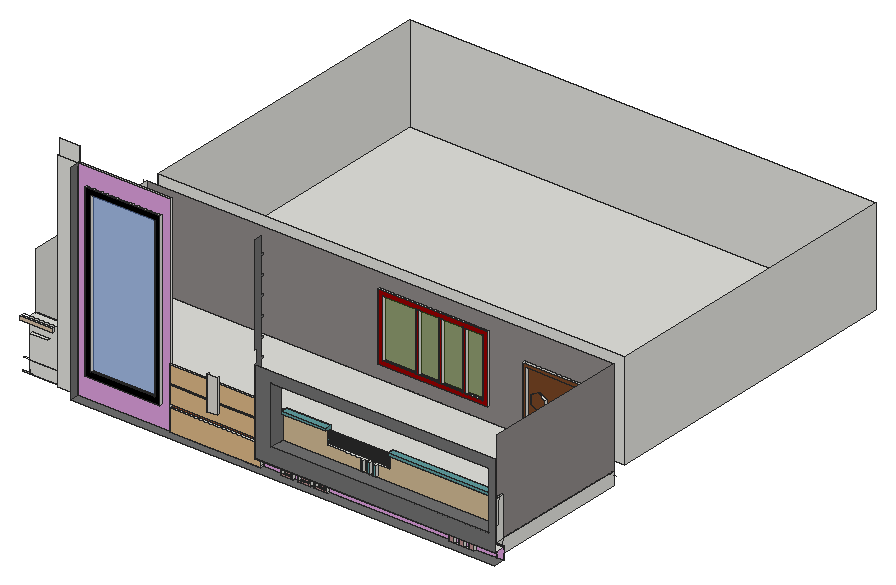
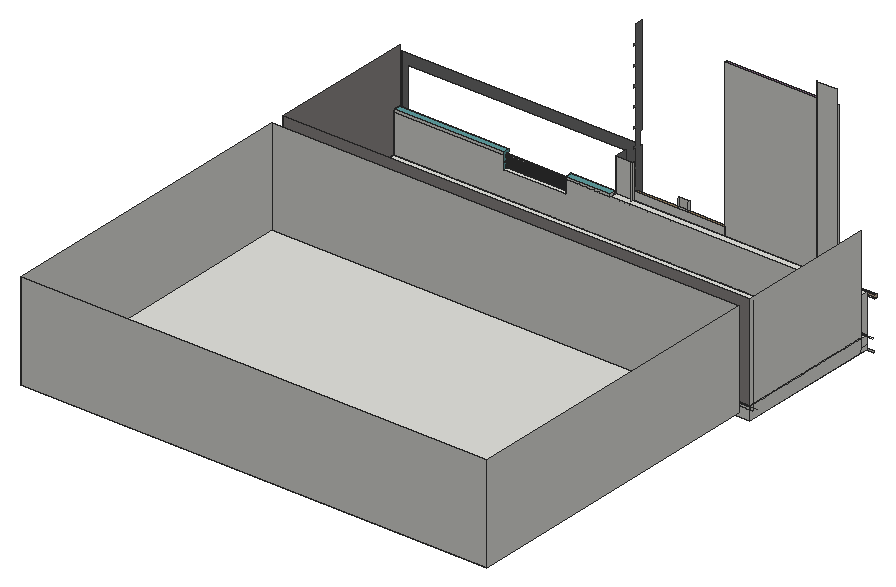
# SketchUp Ruby script. Lengths in inches.
U = 1.inch
M = Sketchup.active_model
def pt(a) = Geom::Point3d.new(a.map { |v| v * U })
def face(e, loops, mat)
  f = e.add_face(loops[0].map { |a| pt(a) })
  loops[1..].each { |l| e.add_face(l.map { |a| pt(a) }).erase! }
  f.material = f.back_material = mat if mat
  f
end
# faces: each face lists its corners as indices into pts; further lists are holes
def faces(e, pts, list, mat = nil) = list.each { |f| face(e, (f[0].is_a?(Array) ? f : [f]).map { |l| l.map { |i| pts[i] } }, mat) }
# xy, xz, yz: faces in a plane at the given z, y or x. An outline is a flat list of corners, or four numbers for a rectangle; further outlines are holes
def ring(l) = l.size == 4 ? [[l[0], l[1]], [l[2], l[1]], [l[2], l[3]], [l[0], l[3]]] : l.each_slice(2).to_a
def flat(e, list, mat, &to3) = list.each { |f| face(e, (f[0].is_a?(Array) ? f : [f]).map { |l| ring(l).map { |u, v| to3.(u, v) } }, mat) }
def xy(e, z, list, mat = nil) = flat(e, list, mat) { |x, y| [x, y, z] }
def xz(e, y, list, mat = nil) = flat(e, list, mat) { |x, z| [x, y, z] }
def yz(e, x, list, mat = nil) = flat(e, list, mat) { |y, z| [x, y, z] }
def lines(e, pts, list) = list.each { |a, b| e.add_line(pt(pts[a]), pt(pts[b])) }
# prism: a flat outline (further loops are holes) pulled along v
def prism(e, loops, v, mat = nil)
  f = face(e, loops, mat); d = Geom::Vector3d.new(v.map { |x| x * U })
  f.pushpull(f.normal.samedirection?(d) ? d.length : -d.length)
end
def box(e, o, s, mat = nil) = prism(e, [[o, [o[0] + s[0], o[1], o[2]], [o[0] + s[0], o[1] + s[1], o[2]], [o[0], o[1] + s[1], o[2]]]], [0, 0, s[2]], mat)
def at(x, y, z, deg = 0) = Geom::Transformation.translation(pt([x, y, z])) * Geom::Transformation.rotation(ORIGIN, Z_AXIS, deg.degrees)
def axes(o, x, y, z) = Geom::Transformation.new([*x, 0, *y, 0, *z, 0, *pt(o).to_a, 1])
def part(name) = M.definitions.add(name)
# library, detail: a bought-in or finely detailed component or shape, given as its bounding box
def library(name, o, s) = part(name).tap { |d| box(d.entities, o, s) }
def detail(e, o, s) = box(e.add_group.entities, o, s)
def put(e, d, t, mat = nil) = e.add_instance(d, t).tap { |i| i.material = mat if mat }
def group(e, t, mat = nil) = e.add_group.tap { |g| g.transformation = t; g.material = mat if mat }.entities
root = M.entities
M.materials.add("[0036_BurlyWood]").color = [222, 184, 135]
M.materials.add("[0042_Sienna]").color = [160, 82, 45]
M.materials.add("[0081_CadetBlue]").color = [95, 158, 160]
M.materials.add("[0119_RosyBrown]").color = [188, 143, 143]
M.materials.add("[0125_Plum]").color = [221, 160, 221]
M.materials.add("[0132_LightGray]").color = [169, 169, 169]
M.materials.add("[0137_Black]").color = [0, 0, 0]
M.materials.add("[Color A07]").color = [153, 0, 0]
M.materials.add("[Color K07]").color = [153, 0, 153]
M.materials.add("[Color M05]").color = [114, 114, 114]
M.materials.add("[Formica Beige]").color = [211, 187, 149]
M.materials.add("[Formica Laminate Light]").color = [213, 189, 164]
M.materials.add("[Stone Marble]").color = [143, 138, 136]
M.materials.add("[Terrazzo Tile Light]").color = [219, 217, 210]
M.materials.add("[Translucent Glass Blue]").color = [100, 149, 237]
M.materials["[Translucent Glass Blue]"].alpha = 0.5
M.materials.add("[Translucent Glass Dark Green]").color = [62, 91, 5]
M.materials["[Translucent Glass Dark Green]"].alpha = 0.5
M.materials.add("[Wood Veneer 01]").color = [120, 70, 37]
xy(root,102.93,[[447.04,325.1,583.06,328.1]])
xy(root,103.875,[[332.83,142.31,447.24,145.31],[687.46,142.43,693.13,142.81],[470.84,142.81,486.83,145.81],[492.01,142.81,508.54,145.81],[511.92,142.81,529.25,145.81],
  [680.89,142.81,687.46,145.81],[687.46,142.81,693.13,145.81],[693.13,142.81,699.69,145.81],[699.69,142.81,705.94,145.81],[705.94,142.81,712.5,145.81],
  [218.42,143.31,332.83,145.31],[193.37,145.81,218.42,146.81],[218.42,145.81,447.24,146.81],[447.24,145.81,467.92,146.81],[467.92,145.81,737.81,146.81],
  [155.81,146.81,737.81,328.1]])
xy(root,103.875,[[218.42,131.81,746.81,131.81,746.81,145.81,712.5,145.81,712.5,142.81,693.13,142.81,693.13,142.43,687.46,142.43,687.46,142.81,680.89,142.81,680.89,145.81,529.25,145.81,529.25,142.81,511.92,142.81,511.92,145.81,508.54,145.81,508.54,142.81,492.01,142.81,492.01,145.81,486.83,145.81,486.83,142.81,470.84,142.81,470.84,145.81,447.24,145.81,447.24,142.31,332.83,142.31,332.83,143.31,218.42,143.31]],"[Color M05]")
xy(root,105.61,[[472.74,142.81,484.93,145.81],[494.18,142.81,506.37,145.81],[514.49,142.81,526.68,145.81]])
xy(root,116.5,[[680.89,142.81,687.46,145.81],[693.13,142.81,699.69,145.81],[705.94,142.81,712.5,145.81]])
xy(root,116.55,[[472.74,142.81,484.93,145.81],[494.18,142.81,506.37,145.81],[514.49,142.81,526.68,145.81]])
xy(root,118.45,[[470.84,142.81,486.83,145.81]])
xy(root,118.6875,[[447.24,131.81,447.37,137.81],[447.37,131.81,447.37,140.81,447.24,140.81,447.24,145.81,492.01,145.81,492.01,142.81,508.54,142.81,508.54,145.81,511.92,145.81,511.92,142.81,529.25,142.81,529.25,145.81,746.74,145.81,746.74,131.81],[746.74,131.81,746.81,145.81],[447.24,137.81,447.37,140.81],[492.01,142.81,508.54,145.81],
  [511.92,142.81,529.25,145.81],[467.92,145.81,737.81,146.81]])
xy(root,120,[[447.24,145.81,467.92,146.81],[155.81,146.81,447.24,148.93],[467.92,146.81,737.81,146.81,737.81,155.81,155.81,155.81,155.81,148.93,447.24,148.93,447.24,147.06,467.92,147.06],[447.24,146.81,467.92,147.06],[155.81,155.81,737.81,155.81,737.81,328.1,698.77,328.1,698.77,325.1,694.77,325.1,694.77,328.1,630.77,328.1,630.77,325.1,626.77,325.1,626.77,328.1,155.81,328.1],
  [626.77,325.1,630.77,328.1],[694.77,325.1,698.77,328.1],[155.81,345.36,737.81,737.81]])
xy(root,121,[[155.81,155.81,737.81,155.81,737.81,328.1,698.77,328.1,698.77,325.1,694.77,325.1,694.77,328.1,630.77,328.1,630.77,325.1,626.77,325.1,626.77,328.1,155.81,328.1]])
xy(root,130.23,[[229.26,140.31,322.76,143.31]])
xy(root,130.625,[[332.83,142.31,447.24,145.31]])
xy(root,134.76,[[332.83,142.31,447.24,145.31]])
xy(root,137.16,[[236.1875,140.31,315.83,143.31]])
xy(root,138.47,[[467.92,131.81,739.66,131.81,739.66,137.81,737.81,146.81,737.81,150.07,467.92,150.07]],"[Color M05]")
xy(root,138.87,[[447.04,325.1,583.06,328.1]])
xy(root,140.25,[[567.0625,147.07,570.68,150.07],[575,147.07,578.62,150.07],[582.375,147.07,585.99,150.07]])
xy(root,144.3,[[452.48,325.1,494.34,328.1],[494.34,325.1,497.5,328.1],[497.5,325.1,522.78,328.1],[522.78,325.1,525.94,328.1],[525.94,325.1,552.97,328.1],
  [552.97,325.1,556.13,328.1],[556.13,325.1,577.62,328.1]])
xy(root,145.14,[[382.48,139.31,394.98,142.31]])
xy(root,152.5625,[[567.0625,147.07,570.68,147.07,570.68,150.07,575,150.07,575,147.07,578.62,147.07,578.62,150.07,582.375,150.07,582.375,147.07,585.99,147.07,585.99,150.07,601.01,150.07,601.01,155.81,523.64,155.81,523.64,150.07,567.0625,150.07]])
xy(root,153.53,[[161.13,141.49,181.44,144.49]])
xy(root,155.4375,[[332.83,142.31,447.24,145.31]])
xy(root,157.83,[[332.83,142.31,447.24,145.31]])
xy(root,162.76,[[146.81,142.49,186.87,144.49]])
xy(root,167.32,[[146.81,142.49,186.87,144.49]])
xy(root,169,[[447.24,145.81,467.92,146.81],[155.81,146.81,447.24,146.81,447.24,147.06,467.92,147.06,467.92,155.81,155.81,155.81],[447.24,146.81,467.92,147.06],[467.92,147.07,523.64,150.07],[601.01,147.07,737.81,150.07]])
xy(root,172,[[467.92,147.07,523.64,155.81],[601.01,147.07,737.81,155.81]],"[0081_CadetBlue]")
xz(root,131.81,[[746.74,118.6875,746.81,223.5]])
xz(root,131.81,[[[447.24,118.6875,746.74,223.5],[467.92,138.47,739.66,210.6875]]],"[Color M05]")
xz(root,139.31,[[382.48,145.14,394.98,186.75]],"[Terrazzo Tile Light]")
xz(root,140.31,[[[229.26,130.23,322.76,341.6],[236.1875,137.16,315.83,334.68]]],"[0137_Black]")
xz(root,142.31,[[382.48,145.14,394.98,145.24],[382.48,145.24,394.98,148.76],[382.48,148.76,394.98,155.4375],[382.48,155.4375,394.98,157.83],[382.48,157.83,394.98,178.5]])
xz(root,142.31,[[332.83,103.875,447.24,130.625],[332.83,134.76,447.24,134.76,447.24,155.4375,394.98,155.4375,394.98,145.14,382.48,145.14,382.48,155.4375,332.83,155.4375],[332.83,157.83,382.48,178.5],[394.98,157.83,447.24,178.5]],"[0036_BurlyWood]")
xz(root,142.49,[[146.81,162.76,186.87,167.32]],"[Formica Laminate Light]")
xz(root,142.81,[[[470.84,103.875,486.83,118.45],[472.74,105.61,484.93,116.55]],[[492.01,103.875,508.54,118.6875],[494.18,105.61,506.37,116.55]],[[511.92,103.875,529.25,118.6875],[514.49,105.61,526.68,116.55]],[680.89,103.875,687.46,116.5],[693.13,103.875,699.69,116.5],
  [705.94,103.875,712.5,116.5]],"[0119_RosyBrown]")
xz(root,143.31,[[193.49,103.875,218.42,363],[[229.26,130.23,322.76,341.6],[236.1875,137.16,315.83,334.68]]])
xz(root,143.31,[[[218.42,103.875,332.83,363],[229.26,130.23,322.76,341.6]]],"[0125_Plum]")
xz(root,143.31,[[236.1875,137.16,315.83,334.68]],"[Translucent Glass Blue]")
xz(root,145.31,[[218.42,103.875,332.83,363],[332.83,103.875,447.24,130.625],[332.83,134.76,447.24,155.4375],[332.83,157.83,447.24,178.5]])
xz(root,145.31,[[332.83,130.625,447.24,134.76],[332.83,155.4375,447.24,157.83]],"[0042_Sienna]")
xz(root,145.81,[[511.92,103.04,529.25,103.875],[492.01,103.44,508.54,103.875],[470.84,103.71,486.83,103.875],[193.37,103.875,218.42,104],[[470.84,103.875,486.83,118.45],[472.74,105.61,484.93,116.55]],
  [[492.01,103.875,508.54,118.6875],[494.18,105.61,506.37,116.55]],[[511.92,103.875,529.25,118.6875],[514.49,105.61,526.68,116.55]],[680.89,103.875,687.46,116.5],[693.13,103.875,699.69,116.5],[705.94,103.875,712.5,116.5],
  [746.74,103.875,746.81,118.6875],[193.37,104,218.42,381.125],[492.01,118.6875,508.54,118.73],[511.92,118.6875,529.25,119.12]])
xz(root,145.81,[[472.74,105.61,484.93,116.55],[494.18,105.61,506.37,116.55],[514.49,105.61,526.68,116.55]],"[0119_RosyBrown]")
xz(root,145.81,[[447.24,103.875,470.84,103.875,470.84,118.45,486.83,118.45,486.83,103.875,492.01,103.875,492.01,118.6875,447.24,118.6875],[529.25,103.875,680.89,103.875,680.89,116.5,687.46,116.5,687.46,103.875,693.13,103.875,693.13,116.5,699.69,116.5,699.69,103.875,705.94,103.875,705.94,116.5,712.5,116.5,712.5,103.875,746.74,103.875,746.74,118.6875,529.25,118.6875]],"[0125_Plum]")
xz(root,145.81,[[508.54,103.875,511.92,118.6875]],"[Color K07]")
xz(root,146.81,[[155.81,103.875,193.37,104],[193.37,103.875,447.24,103.875,447.24,120,155.81,120,155.81,104,193.37,104],[447.24,103.875,467.92,108.75],[467.92,103.875,737.81,118.6875],[146.81,104,155.81,105.875],
  [447.24,108.75,467.92,118.6875],[447.24,118.6875,467.92,120],[467.92,118.6875,737.81,120],[155.81,120,447.24,169],[447.24,169,467.92,210.6875]])
xz(root,147.07,[[567.0625,140.25,570.68,152.5625],[575,140.25,578.62,152.5625],[582.375,140.25,585.99,152.5625],[467.92,169,523.64,172],[601.01,169,737.81,172]],"[0081_CadetBlue]")
xz(root,150.07,[[467.92,138.47,737.81,138.47,737.81,169,601.01,169,601.01,152.5625,585.99,152.5625,585.99,140.25,582.375,140.25,582.375,152.5625,578.62,152.5625,578.62,140.25,575,140.25,575,152.5625,570.68,152.5625,570.68,140.25,567.0625,140.25,567.0625,152.5625,523.64,152.5625,523.64,169,467.92,169]],"[Formica Beige]")
xz(root,155.81,[[155.81,108.75,737.81,120],[155.81,120,737.81,121],[155.81,121,155.81,169,523.64,169,523.64,152.5625,601.01,152.5625,601.01,169,737.81,169,737.81,121],[467.92,169,523.64,172],[601.01,169,737.81,172]])
xz(root,325.1,[[626.77,120,630.77,121],[694.77,120,698.77,121]])
xz(root,325.1,[[[447.04,138.87,583.06,222.93],[452.48,144.3,577.62,217.49]],[494.34,144.3,497.5,217.49],[522.78,144.3,525.94,217.49],[552.97,144.3,556.13,217.49]],"[Color A07]")
xz(root,325.1,[[626.77,121,630.77,121,630.77,200,694.77,200,694.77,121,698.77,121,698.77,204,626.77,204],[645.84,156.08,654.56,161.11,654.56,171.18,645.84,176.21,637.13,171.18,637.13,161.11]],"[Wood Veneer 01]")
xz(root,328.1,[[155.81,103.875,626.77,116],[626.77,103.875,630.77,116],[630.77,103.875,694.77,120],[694.77,103.875,698.77,116],[698.77,103.875,737.81,116],
  [151.81,116,155.81,120],[155.81,116,626.77,120],[626.77,116,630.77,120],[694.77,116,698.77,120],[698.77,116,737.81,120],
  [155.81,120,626.77,121],[626.77,120,626.77,204,698.77,204,698.77,120,694.77,120,694.77,200,630.77,200,630.77,120],[630.77,120,694.77,121],[698.77,120,737.81,121],[[447.04,138.87,583.06,222.93],[452.48,144.3,577.62,217.49]],
  [494.34,144.3,497.5,217.49],[522.78,144.3,525.94,217.49],[552.97,144.3,556.13,217.49],[645.84,156.08,637.13,161.11,637.13,171.18,645.84,176.21,654.56,171.18,654.56,161.11]])
xz(root,328.1,[[[155.81,121,626.77,121,626.77,204,698.77,204,698.77,121,737.81,121,737.81,240,155.81,240],[447.04,138.87,583.06,222.93]]],"[Stone Marble]")
xz(root,328.1,[[452.48,144.3,494.34,217.49],[497.5,144.3,522.78,217.49],[525.94,144.3,552.97,217.49],[556.13,144.3,577.62,217.49]],"[Translucent Glass Dark Green]")
xz(root,328.1,[[[630.77,121,694.77,200],[645.84,156.08,637.13,161.11,637.13,171.18,645.84,176.21,654.56,171.18,654.56,161.11]]],"[Wood Veneer 01]")
xz(root,345.36,[[155.81,120,737.81,240]])
xz(root,737.81,[[155.81,120,737.81,240]])
yz(root,155.81,[[146.81,103.875,155.81,108.75],[155.81,103.875,328.1,120],[155.81,120,328.1,121],[345.36,120,737.81,240],[155.81,121,328.1,240]])
yz(root,186.87,[[142.49,162.76,144.49,167.32]])
yz(root,193.37,[[145.81,103.875,146.81,104]])
yz(root,218.42,[[143.31,103.875,144.49,363],[144.49,103.875,145.31,104],[144.49,104,145.31,363],[145.31,104,145.81,381.125]])
yz(root,218.42,[[131.81,103.875,143.31,103.875,143.31,363,145.31,363,145.31,363.3125,137.81,363.3125,137.81,363,131.81,363]],"[Color M05]")
yz(root,229.26,[[140.31,130.23,143.31,341.6]])
yz(root,236.1875,[[140.31,137.16,143.31,334.68]])
yz(root,315.83,[[140.31,137.16,143.31,334.68]])
yz(root,322.76,[[140.31,130.23,143.31,341.6]])
yz(root,332.83,[[142.31,103.875,143.31,130.625],[143.31,103.875,145.31,130.625],[143.31,130.625,145.31,134.76],[142.31,134.76,143.31,155.4375],[143.31,134.76,145.31,155.4375],
  [143.31,155.4375,145.31,157.83],[142.31,157.83,143.31,178.5],[143.31,157.83,145.31,178.5]])
yz(root,382.48,[[139.31,145.14,142.31,186.75]])
yz(root,394.98,[[139.31,145.14,142.31,186.75]])
yz(root,447.04,[[325.1,138.87,328.1,222.93]])
yz(root,447.24,[[142.31,103.875,145.31,105.875],[145.31,103.875,145.81,105.875],[145.81,103.875,146.81,105.875],[142.31,105.875,145.31,118.6875],[145.31,105.875,145.81,118.6875],
  [145.81,105.875,146.81,120],[142.31,118.6875,145.31,119.3125],[145.31,118.6875,145.81,120],[142.31,119.3125,145.31,120],[142.31,120,145.31,130.625],
  [145.31,120,145.81,120,145.81,169,146.81,169,146.81,210.6875,145.31,210.6875],[145.81,120,146.81,169],[146.81,120,147.06,169],[147.06,120,148.93,120,148.93,210.6875,146.81,210.6875,146.81,169,147.06,169],[142.31,134.76,145.31,144.125],
  [142.31,144.125,145.31,155.4375],[142.31,157.83,145.31,167.1875],[142.31,167.1875,145.31,178.5]])
yz(root,447.24,[[131.81,118.6875,131.81,223.5,134.81,223.5,134.81,240,131.81,240,131.81,363,142.31,363,142.31,342.33,145.31,342.33,145.31,339.9375,142.31,339.9375,142.31,319.26,145.31,319.26,145.31,316.875,142.31,316.875,142.31,296.2,145.31,296.2,145.31,293.8125,142.31,293.8125,142.31,273.14,145.31,273.14,145.31,270.75,142.31,270.75,142.31,250.08,145.31,250.08,145.31,247.6875,142.31,247.6875,142.31,227.01,145.31,227.01,145.31,224.625,142.31,224.625,142.31,203.95,145.31,203.95,145.31,201.5625,142.31,201.5625,142.31,180.89,145.31,180.89,145.31,178.5,142.31,178.5,142.31,157.83,145.31,157.83,145.31,155.4375,142.31,155.4375,142.31,134.76,145.31,134.76,145.31,130.625,142.31,130.625,142.31,118.6875]],"[Color M05]")
yz(root,447.37,[[137.81,118.6875,140.81,120,140.81,118.6875]])
yz(root,452.48,[[325.1,144.3,328.1,217.49]])
yz(root,467.92,[[145.81,118.6875,146.81,120],[145.81,120,146.81,138.47],[146.81,120,147.06,138.47],[147.07,169,150.07,172],[150.07,169,155.81,172]])
yz(root,467.92,[[131.81,138.47,150.07,138.47,150.07,169,146.81,169,146.81,210.6875,131.81,210.6875]],"[Color M05]")
yz(root,470.84,[[142.81,103.71,145.81,103.875],[142.81,103.875,145.81,118.45]])
yz(root,472.74,[[142.81,105.61,145.81,116.55]])
yz(root,484.93,[[142.81,105.61,145.81,116.55]])
yz(root,486.83,[[142.81,103.71,145.81,103.875],[142.81,103.875,145.81,118.45]])
yz(root,492.01,[[142.81,103.44,145.81,103.875],[142.81,103.875,145.81,118.6875]])
yz(root,494.18,[[142.81,105.61,145.81,116.55]])
yz(root,494.34,[[325.1,144.3,328.1,217.49]])
yz(root,497.5,[[325.1,144.3,328.1,217.49]])
yz(root,506.37,[[142.81,105.61,145.81,116.55]])
yz(root,508.54,[[142.81,103.44,145.81,103.875],[142.81,103.875,145.81,118.6875]])
yz(root,511.92,[[142.81,103.04,145.81,103.875],[142.81,103.875,145.81,118.6875]])
yz(root,514.49,[[142.81,105.61,145.81,116.55]])
yz(root,522.78,[[325.1,144.3,328.1,217.49]])
yz(root,523.64,[[[150.07,152.5625,155.81,152.5625,155.81,172,147.07,172,147.07,169,150.07,169],[151.76,165.5,151.32,165.5625,150.91,165.73,150.5625,166,150.29,166.35,150.125,166.75,150.07,167.19,150.125,167.63,150.29,168.03,150.5625,168.38,150.91,168.65,151.32,168.82,151.76,168.88,152.19,168.82,152.6,168.65,152.95,168.38,153.22,168.03,153.39,167.63,153.44,167.19,153.39,166.75,153.22,166.35,152.95,166,152.6,165.73,152.19,165.5625],[151.76,159.44,151.32,159.5,150.91,159.67,150.5625,159.94,150.29,160.28,150.125,160.69,150.07,161.13,150.125,161.57,150.29,161.97,150.5625,162.32,150.91,162.59,151.32,162.76,151.76,162.82,152.19,162.76,152.6,162.59,152.95,162.32,153.22,161.97,153.39,161.57,153.44,161.13,153.39,160.69,153.22,160.28,152.95,159.94,152.6,159.67,152.19,159.5],[151.76,154.13,151.32,154.1875,150.91,154.35,150.5625,154.62,150.29,154.97,150.125,155.38,150.07,155.82,150.125,156.25,150.29,156.66,150.5625,157.01,150.91,157.28,151.32,157.45,151.76,157.5,152.19,157.45,152.6,157.28,152.95,157.01,153.22,156.66,153.39,156.25,153.44,155.82,153.39,155.38,153.22,154.97,152.95,154.62,152.6,154.35,152.19,154.1875]]],"[0081_CadetBlue]")
yz(root,525.94,[[325.1,144.3,328.1,217.49]])
yz(root,526.68,[[142.81,105.61,145.81,116.55]])
yz(root,529.25,[[142.81,103.04,145.81,103.875],[142.81,103.875,145.81,118.6875]])
yz(root,552.97,[[325.1,144.3,328.1,217.49]])
yz(root,556.13,[[325.1,144.3,328.1,217.49]])
yz(root,567.0625,[[147.07,140.25,150.07,152.5625]])
yz(root,570.68,[[147.07,140.25,150.07,152.5625]])
yz(root,575,[[147.07,140.25,150.07,152.5625]])
yz(root,577.62,[[325.1,144.3,328.1,217.49]])
yz(root,578.62,[[147.07,140.25,150.07,152.5625]])
yz(root,582.375,[[147.07,140.25,150.07,152.5625]])
yz(root,583.06,[[325.1,138.87,328.1,222.93]])
yz(root,585.99,[[147.07,140.25,150.07,152.5625]])
yz(root,600.64,[[151.76,154.13,152.19,154.1875,152.6,154.35,152.95,154.62,153.22,154.97,153.39,155.38,153.44,155.82,153.39,156.25,153.22,156.66,152.95,157.01,152.6,157.28,152.19,157.45,151.76,157.5,151.32,157.45,150.91,157.28,150.5625,157.01,150.29,156.66,150.125,156.25,150.07,155.82,150.125,155.38,150.29,154.97,150.5625,154.62,150.91,154.35,151.32,154.1875]])
yz(root,601.01,[[[150.07,152.5625,150.07,169,147.07,169,147.07,172,155.81,172,155.81,152.5625],[151.76,165.5,152.19,165.5625,152.6,165.73,152.95,166,153.22,166.35,153.39,166.75,153.44,167.19,153.39,167.63,153.22,168.03,152.95,168.38,152.6,168.65,152.19,168.82,151.76,168.88,151.32,168.82,150.91,168.65,150.5625,168.38,150.29,168.03,150.125,167.63,150.07,167.19,150.125,166.75,150.29,166.35,150.5625,166,150.91,165.73,151.32,165.5625],[151.76,159.44,152.19,159.5,152.6,159.67,152.95,159.94,153.22,160.28,153.39,160.69,153.44,161.13,153.39,161.57,153.22,161.97,152.95,162.32,152.6,162.59,152.19,162.76,151.76,162.82,151.32,162.76,150.91,162.59,150.5625,162.32,150.29,161.97,150.125,161.57,150.07,161.13,150.125,160.69,150.29,160.28,150.5625,159.94,150.91,159.67,151.32,159.5]]],"[0081_CadetBlue]")
yz(root,626.77,[[325.1,120,328.1,121],[325.1,121,328.1,204]])
yz(root,630.77,[[325.1,120,328.1,121],[325.1,121,328.1,200]])
yz(root,637.13,[[325.1,161.11,328.1,171.18]])
yz(root,654.56,[[325.1,161.11,328.1,171.18]])
yz(root,680.89,[[142.81,103.875,145.81,116.5]],"[0119_RosyBrown]")
yz(root,687.46,[[142.81,103.875,145.81,116.5]])
yz(root,693.13,[[142.81,103.875,145.81,116.5]],"[0119_RosyBrown]")
yz(root,694.77,[[325.1,120,328.1,121],[325.1,121,328.1,200]])
yz(root,698.77,[[325.1,120,328.1,121],[325.1,121,328.1,204]])
yz(root,699.69,[[142.81,103.875,145.81,116.5]])
yz(root,705.94,[[142.81,103.875,145.81,116.5]],"[0119_RosyBrown]")
yz(root,712.5,[[142.81,103.875,145.81,116.5]])
yz(root,737.81,[[146.81,103.875,155.81,108.75],[155.81,103.875,328.1,120],[146.81,108.75,155.81,120],[146.81,120,146.81,138.47,150.07,138.47,150.07,169,155.81,169,155.81,120],[155.81,120,328.1,121],
  [345.36,120,737.81,240],[146.81,138.47,150.07,169],[147.07,169,150.07,172],[150.07,169,155.81,172]])
yz(root,737.81,[[155.81,121,155.81,172,147.07,172,147.07,169,146.81,169,146.81,240,328.1,240,328.1,121]],"[Stone Marble]")
p = [[523.64,151.32,154.1875],[523.64,151.76,154.13],[600.64,151.76,154.13],[600.64,151.32,154.1875],[523.64,152.19,154.1875],[600.64,152.19,154.1875],
  [523.64,150.91,154.35],[600.64,150.91,154.35],[523.64,152.6,154.35],[600.64,152.6,154.35],[523.64,150.5625,154.62],[600.64,150.5625,154.62],
  [523.64,152.95,154.62],[600.64,152.95,154.62],[523.64,150.29,154.97],[600.64,150.29,154.97],[523.64,153.22,154.97],[600.64,153.22,154.97],
  [523.64,150.125,155.38],[600.64,150.125,155.38],[523.64,153.39,155.38],[600.64,153.39,155.38],[523.64,150.07,155.82],[600.64,150.07,155.82],
  [523.64,153.44,155.82],[600.64,153.44,155.82],[523.64,150.125,156.25],[600.64,150.125,156.25],[523.64,153.39,156.25],[600.64,153.39,156.25],
  [637.13,328.1,161.11],[645.84,328.1,156.08],[645.84,325.1,156.08],[637.13,325.1,161.11],[654.56,328.1,161.11],[654.56,325.1,161.11],
  [523.64,150.29,156.66],[600.64,150.29,156.66],[523.64,153.22,156.66],[600.64,153.22,156.66],[523.64,150.5625,157.01],[600.64,150.5625,157.01],
  [523.64,152.95,157.01],[600.64,152.95,157.01],[523.64,150.91,157.28],[600.64,150.91,157.28],[523.64,152.6,157.28],[600.64,152.6,157.28],
  [523.64,151.32,157.45],[600.64,151.32,157.45],[523.64,152.19,157.45],[600.64,152.19,157.45],[523.64,151.76,157.5],[600.64,151.76,157.5],
  [523.64,151.32,159.5],[523.64,151.76,159.44],[601.01,151.76,159.44],[601.01,151.32,159.5],[523.64,152.19,159.5],[601.01,152.19,159.5],
  [523.64,150.91,159.67],[601.01,150.91,159.67],[523.64,152.6,159.67],[601.01,152.6,159.67],[523.64,150.5625,159.94],[601.01,150.5625,159.94],
  [523.64,152.95,159.94],[601.01,152.95,159.94],[523.64,150.29,160.28],[601.01,150.29,160.28],[523.64,153.22,160.28],[601.01,153.22,160.28],
  [523.64,150.125,160.69],[601.01,150.125,160.69],[523.64,153.39,160.69],[601.01,153.39,160.69],[523.64,150.07,161.13],[601.01,150.07,161.13],
  [523.64,153.44,161.13],[601.01,153.44,161.13],[523.64,150.125,161.57],[601.01,150.125,161.57],[523.64,153.39,161.57],[601.01,153.39,161.57],
  [523.64,150.29,161.97],[601.01,150.29,161.97],[523.64,153.22,161.97],[601.01,153.22,161.97],[523.64,150.5625,162.32],[601.01,150.5625,162.32],
  [523.64,152.95,162.32],[601.01,152.95,162.32],[523.64,150.91,162.59],[601.01,150.91,162.59],[523.64,152.6,162.59],[601.01,152.6,162.59],
  [523.64,151.32,162.76],[601.01,151.32,162.76],[523.64,152.19,162.76],[601.01,152.19,162.76],[523.64,151.76,162.82],[601.01,151.76,162.82],
  [523.64,151.32,165.5625],[523.64,151.76,165.5],[601.01,151.76,165.5],[601.01,151.32,165.5625],[523.64,152.19,165.5625],[601.01,152.19,165.5625],
  [523.64,150.91,165.73],[601.01,150.91,165.73],[523.64,152.6,165.73],[601.01,152.6,165.73],[523.64,150.5625,166],[601.01,150.5625,166],
  [523.64,152.95,166],[601.01,152.95,166],[523.64,150.29,166.35],[601.01,150.29,166.35],[523.64,153.22,166.35],[601.01,153.22,166.35],
  [523.64,150.125,166.75],[601.01,150.125,166.75],[523.64,153.39,166.75],[601.01,153.39,166.75],[523.64,150.07,167.19],[601.01,150.07,167.19],
  [523.64,153.44,167.19],[601.01,153.44,167.19],[523.64,150.125,167.63],[601.01,150.125,167.63],[523.64,153.39,167.63],[601.01,153.39,167.63],
  [523.64,150.29,168.03],[601.01,150.29,168.03],[523.64,153.22,168.03],[601.01,153.22,168.03],[523.64,150.5625,168.38],[601.01,150.5625,168.38],
  [523.64,152.95,168.38],[601.01,152.95,168.38],[523.64,150.91,168.65],[601.01,150.91,168.65],[523.64,152.6,168.65],[601.01,152.6,168.65],
  [523.64,151.32,168.82],[601.01,151.32,168.82],[523.64,152.19,168.82],[601.01,152.19,168.82],[523.64,151.76,168.88],[601.01,151.76,168.88],
  [645.84,328.1,176.21],[637.13,328.1,171.18],[637.13,325.1,171.18],[645.84,325.1,176.21],[654.56,328.1,171.18],[654.56,325.1,171.18],
  [151.81,328.1,120],[146.81,328.1,120],[151.81,328.1,240],[737.81,328.1,116],[741.81,328.1,116],[155.81,146.81,169],
  [146.81,146.81,169],[155.81,146.81,120],[146.81,146.81,120],[630.77,325.1,120],[630.77,325.1,103.875],[737.81,146.81,120],
  [746.81,146.81,120],[467.92,146.81,108.75],[467.92,145.81,108.75],[467.92,137.81,120],[467.92,145.81,120],[447.37,137.81,120],
  [447.37,140.81,120],[447.24,140.81,120],[737.81,146.81,108.75],[746.81,146.81,108.75],[737.81,146.81,103.875],[746.81,146.81,103.875],
  [737.81,146.81,118.6875],[746.81,146.81,118.6875],[698.77,325.1,120],[698.77,325.1,103.875],[694.77,325.1,120],[694.77,325.1,103.875],
  [626.77,325.1,120],[626.77,325.1,103.875],[155.81,148.93,120],[146.81,148.93,120],[529.25,142.81,103.04],[529.25,131.81,103.04]]
faces(root,p,[[0,1,2,3],[1,4,5,2],[6,0,3,7],[4,8,9,5],[10,6,7,11],[8,12,13,9],[14,10,11,15],[12,16,17,13],
  [18,14,15,19],[16,20,21,17],[22,18,19,23],[20,24,25,21],[26,22,23,27],[24,28,29,25],[36,26,27,37],[28,38,39,29],
  [40,36,37,41],[38,42,43,39],[44,40,41,45],[42,46,47,43],[48,44,45,49],[46,50,51,47],[52,48,49,53],[50,52,53,51],
  [54,55,56,57],[55,58,59,56],[60,54,57,61],[58,62,63,59],[64,60,61,65],[62,66,67,63],[68,64,65,69],[66,70,71,67],
  [72,68,69,73],[70,74,75,71],[76,72,73,77],[74,78,79,75],[80,76,77,81],[78,82,83,79],[84,80,81,85],[82,86,87,83],
  [88,84,85,89],[86,90,91,87],[92,88,89,93],[90,94,95,91],[96,92,93,97],[94,98,99,95],[100,96,97,101],[98,100,101,99],
  [102,103,104,105],[103,106,107,104],[108,102,105,109],[106,110,111,107],[112,108,109,113],[110,114,115,111],[116,112,113,117],[114,118,119,115],
  [120,116,117,121],[118,122,123,119],[124,120,121,125],[122,126,127,123],[128,124,125,129],[126,130,131,127],[132,128,129,133],[130,134,135,131],
  [136,132,133,137],[134,138,139,135],[140,136,137,141],[138,142,143,139],[144,140,141,145],[142,146,147,143],[148,144,145,149],[146,148,149,147]],"[0132_LightGray]")
faces(root,p,[[30,31,32,33],[31,34,35,32],[150,151,152,153],[154,150,153,155]])
lines(root,p,[[156,157],[158,156],[159,160],[161,162],[163,164],[165,166],[167,168],[169,170],[171,172],[173,174],[175,174],[176,177],
  [178,179],[180,181],[182,183],[184,185],[186,187],[188,189],[190,191]])
